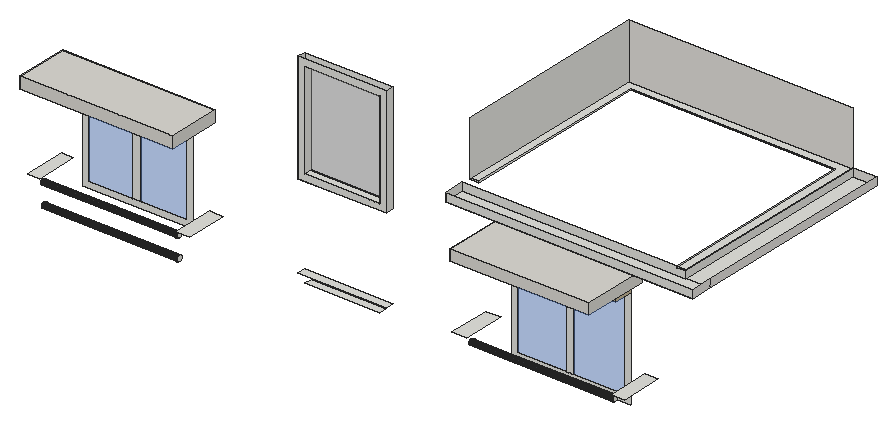
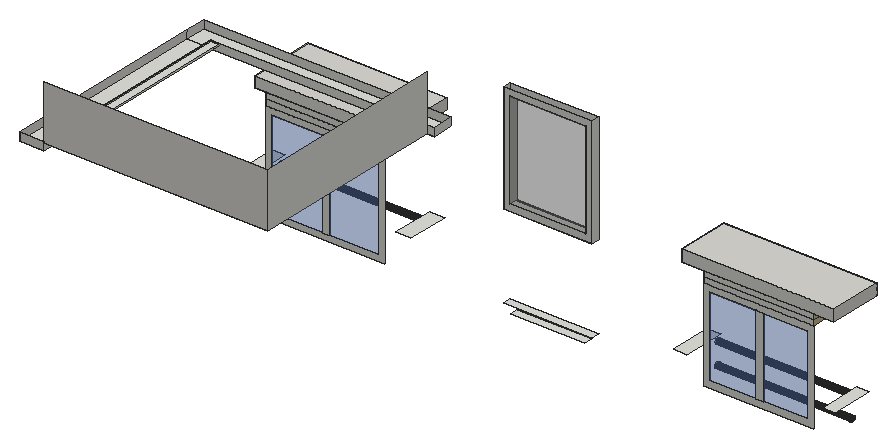
# SketchUp Ruby script. Lengths in inches.
U = 1.inch
M = Sketchup.active_model
def pt(a) = Geom::Point3d.new(a.map { |v| v * U })
def face(e, loops, mat)
  f = e.add_face(loops[0].map { |a| pt(a) })
  loops[1..].each { |l| e.add_face(l.map { |a| pt(a) }).erase! }
  f.material = f.back_material = mat if mat
  f
end
# faces: each face lists its corners as indices into pts; further lists are holes
def faces(e, pts, list, mat = nil) = list.each { |f| face(e, (f[0].is_a?(Array) ? f : [f]).map { |l| l.map { |i| pts[i] } }, mat) }
# xy, xz, yz: faces in a plane at the given z, y or x. An outline is a flat list of corners, or four numbers for a rectangle; further outlines are holes
def ring(l) = l.size == 4 ? [[l[0], l[1]], [l[2], l[1]], [l[2], l[3]], [l[0], l[3]]] : l.each_slice(2).to_a
def flat(e, list, mat, &to3) = list.each { |f| face(e, (f[0].is_a?(Array) ? f : [f]).map { |l| ring(l).map { |u, v| to3.(u, v) } }, mat) }
def xy(e, z, list, mat = nil) = flat(e, list, mat) { |x, y| [x, y, z] }
def xz(e, y, list, mat = nil) = flat(e, list, mat) { |x, z| [x, y, z] }
def yz(e, x, list, mat = nil) = flat(e, list, mat) { |y, z| [x, y, z] }
def lines(e, pts, list) = list.each { |a, b| e.add_line(pt(pts[a]), pt(pts[b])) }
# prism: a flat outline (further loops are holes) pulled along v
def prism(e, loops, v, mat = nil)
  f = face(e, loops, mat); d = Geom::Vector3d.new(v.map { |x| x * U })
  f.pushpull(f.normal.samedirection?(d) ? d.length : -d.length)
end
def box(e, o, s, mat = nil) = prism(e, [[o, [o[0] + s[0], o[1], o[2]], [o[0] + s[0], o[1] + s[1], o[2]], [o[0], o[1] + s[1], o[2]]]], [0, 0, s[2]], mat)
def at(x, y, z, deg = 0) = Geom::Transformation.translation(pt([x, y, z])) * Geom::Transformation.rotation(ORIGIN, Z_AXIS, deg.degrees)
def axes(o, x, y, z) = Geom::Transformation.new([*x, 0, *y, 0, *z, 0, *pt(o).to_a, 1])
def part(name) = M.definitions.add(name)
# library, detail: a bought-in or finely detailed component or shape, given as its bounding box
def library(name, o, s) = part(name).tap { |d| box(d.entities, o, s) }
def detail(e, o, s) = box(e.add_group.entities, o, s)
def put(e, d, t, mat = nil) = e.add_instance(d, t).tap { |i| i.material = mat if mat }
def group(e, t, mat = nil) = e.add_group.tap { |g| g.transformation = t; g.material = mat if mat }.entities
root = M.entities
M.materials.add("[Color M07]").color = [58, 58, 58]
M.materials.add("[Formica Laminate Dark]").color = [50, 53, 60]
M.materials.add("[Quartz Light Brown]").color = [199, 184, 152]
M.materials.add("[Terrazzo Tile Accent]").color = [224, 221, 217]
M.materials.add("[Terrazzo Tile Light]").color = [219, 217, 210]
M.materials.add("[Translucent Glass Blue]").color = [85, 126, 201]
M.materials["[Translucent Glass Blue]"].alpha = 0.5
M.materials.add("[Translucent Glass Gray]").color = [128, 128, 128]
M.materials["[Translucent Glass Gray]"].alpha = 0.5
xy(root,492.32,[[183.4,109.54,226.8,114.1]])
xy(root,496.3125,[[179.41,109.54,230.79,114.1]])
xy(root,503.49,[[103.3,91.47,103.56,91.5,103.8,91.6,104.01,91.76,104.16,91.97,104.26,92.21,104.3,92.47,104.26,92.73,104.16,92.97,104.01,93.18,103.8,93.33,103.56,93.43,103.3,93.47,103.04,93.43,102.8,93.33,102.59,93.18,102.43,92.97,102.33,92.73,102.3,92.47,102.33,92.21,102.43,91.97,102.59,91.76,102.8,91.6,103.04,91.5]])
xy(root,503.62,[[67.24,91.47,67.49,91.5,67.74,91.6,67.94,91.76,68.1,91.97,68.2,92.21,68.24,92.47,68.2,92.73,68.1,92.97,67.94,93.18,67.74,93.33,67.49,93.43,67.24,93.47,66.98,93.43,66.74,93.33,66.53,93.18,66.37,92.97,66.27,92.73,66.24,92.47,66.27,92.21,66.37,91.97,66.53,91.76,66.74,91.6,66.98,91.5]])
xy(root,504.05,[[108.86,91.47,109.12,91.5,109.36,91.6,109.57,91.76,109.73,91.97,109.83,92.21,109.86,92.47,109.83,92.73,109.73,92.97,109.57,93.18,109.36,93.33,109.12,93.43,108.86,93.47,108.6,93.43,108.36,93.33,108.15,93.18,107.99,92.97,107.89,92.73,107.86,92.47,107.89,92.21,107.99,91.97,108.15,91.76,108.36,91.6,108.6,91.5]])
xy(root,504.12,[[72.86,91.47,73.12,91.5,73.36,91.6,73.57,91.76,73.73,91.97,73.83,92.21,73.86,92.47,73.83,92.73,73.73,92.97,73.57,93.18,73.36,93.33,73.12,93.43,72.86,93.47,72.6,93.43,72.36,93.33,72.15,93.18,71.99,92.97,71.89,92.73,71.86,92.47,71.89,92.21,71.99,91.97,72.15,91.76,72.36,91.6,72.6,91.5]])
xy(root,504.18,[[78.17,91.47,78.43,91.5,78.67,91.6,78.88,91.76,79.04,91.97,79.14,92.21,79.17,92.47,79.14,92.73,79.04,92.97,78.88,93.18,78.67,93.33,78.43,93.43,78.17,93.47,77.91,93.43,77.67,93.33,77.47,93.18,77.31,92.97,77.21,92.73,77.17,92.47,77.21,92.21,77.31,91.97,77.47,91.76,77.67,91.6,77.91,91.5]])
xy(root,504.3,[[61.92,91.47,62.18,91.5,62.42,91.6,62.63,91.76,62.79,91.97,62.89,92.21,62.92,92.47,62.89,92.73,62.79,92.97,62.63,93.18,62.42,93.33,62.18,93.43,61.92,93.47,61.66,93.43,61.42,93.33,61.22,93.18,61.06,92.97,60.96,92.73,60.92,92.47,60.96,92.21,61.06,91.97,61.22,91.76,61.42,91.6,61.66,91.5]])
xy(root,504.43,[[97.92,91.47,98.18,91.5,98.42,91.6,98.63,91.76,98.79,91.97,98.89,92.21,98.92,92.47,98.89,92.73,98.79,92.97,98.63,93.18,98.42,93.33,98.18,93.43,97.92,93.47,97.66,93.43,97.42,93.33,97.22,93.18,97.06,92.97,96.96,92.73,96.92,92.47,96.96,92.21,97.06,91.97,97.22,91.76,97.42,91.6,97.66,91.5]])
xy(root,504.49,[[52.05,91.47,52.31,91.5,52.55,91.6,52.76,91.76,52.91,91.97,53.01,92.21,53.05,92.47,53.01,92.73,52.91,92.97,52.76,93.18,52.55,93.33,52.31,93.43,52.05,93.47,51.79,93.43,51.55,93.33,51.34,93.18,51.18,92.97,51.08,92.73,51.05,92.47,51.08,92.21,51.18,91.97,51.34,91.76,51.55,91.6,51.79,91.5]])
xy(root,504.67,[[92.55,91.47,92.81,91.5,93.05,91.6,93.26,91.76,93.41,91.97,93.51,92.21,93.55,92.47,93.51,92.73,93.41,92.97,93.26,93.18,93.05,93.33,92.81,93.43,92.55,93.47,92.29,93.43,92.05,93.33,91.84,93.18,91.68,92.97,91.58,92.73,91.55,92.47,91.58,92.21,91.68,91.97,91.84,91.76,92.05,91.6,92.29,91.5],[115.11,91.47,115.37,91.5,115.61,91.6,115.82,91.76,115.98,91.97,116.08,92.21,116.11,92.47,116.08,92.73,115.98,92.97,115.82,93.18,115.61,93.33,115.37,93.43,115.11,93.47,114.85,93.43,114.61,93.33,114.4,93.18,114.24,92.97,114.14,92.73,114.11,92.47,114.14,92.21,114.24,91.97,114.4,91.76,114.61,91.6,114.85,91.5],[120.49,91.47,120.74,91.5,120.99,91.6,121.19,91.76,121.35,91.97,121.45,92.21,121.49,92.47,121.45,92.73,121.35,92.97,121.19,93.18,120.99,93.33,120.74,93.43,120.49,93.47,120.23,93.43,119.99,93.33,119.78,93.18,119.62,92.97,119.52,92.73,119.49,92.47,119.52,92.21,119.62,91.97,119.78,91.76,119.99,91.6,120.23,91.5]])
xy(root,504.8,[[84.85,90.875,85.25,90.93,85.625,91.08,85.95,91.33,86.2,91.66,86.35,92.03,86.41,92.4375,86.35,92.84,86.2,93.22,85.95,93.54,85.625,93.79,85.25,93.95,84.85,94,84.44,93.95,84.0625,93.79,83.74,93.54,83.49,93.22,83.34,92.84,83.28,92.4375,83.34,92.03,83.49,91.66,83.74,91.33,84.0625,91.08,84.44,90.93]])
xy(root,505.01,[[47.49,91.47,47.74,91.5,47.99,91.6,48.19,91.76,48.35,91.97,48.45,92.21,48.49,92.47,48.45,92.73,48.35,92.97,48.19,93.18,47.99,93.33,47.85,93.39,47.12,93.39,46.99,93.33,46.78,93.18,46.62,92.97,46.52,92.73,46.49,92.47,46.52,92.21,46.62,91.97,46.78,91.76,46.99,91.6,47.23,91.5],[56.74,91.47,56.99,91.5,57.24,91.6,57.44,91.76,57.6,91.97,57.7,92.21,57.74,92.47,57.7,92.73,57.6,92.97,57.44,93.18,57.24,93.33,57.1,93.39,56.37,93.39,56.24,93.33,56.03,93.18,55.87,92.97,55.77,92.73,55.74,92.47,55.77,92.21,55.87,91.97,56.03,91.76,56.24,91.6,56.48,91.5],[47.12,93.39,47.85,93.39,47.74,93.43,47.49,93.47,47.23,93.43],[56.37,93.39,57.1,93.39,56.99,93.43,56.74,93.47,56.48,93.43]])
xy(root,506.99,[[38.09,89.73,44.94,114.1],[124.21,89.73,132.15,114.1]])
xy(root,507.16,[[359.09,91.9,359.32,91.93,359.53,92.02,359.71,92.16,359.85,92.34,359.9375,92.55,359.97,92.78,359.9375,93.01,359.85,93.22,359.71,93.4,359.53,93.54,359.32,93.625,359.09,93.65,358.86,93.625,358.65,93.54,358.47,93.4,358.33,93.22,358.25,93.01,358.22,92.78,358.25,92.55,358.33,92.34,358.47,92.16,358.65,92.02,358.86,91.93]])
xy(root,507.22,[[300.4,91.9,300.63,91.93,300.84,92.02,301.02,92.16,301.16,92.34,301.25,92.55,301.28,92.78,301.25,93.01,301.16,93.22,301.02,93.4,300.84,93.54,300.63,93.625,300.4,93.65,300.18,93.625,299.97,93.54,299.78,93.4,299.65,93.22,299.56,93.01,299.53,92.78,299.56,92.55,299.65,92.34,299.78,92.16,299.97,92.02,300.18,91.93]])
xy(root,507.41,[[305.59,91.9,305.82,91.93,306.03,92.02,306.21,92.16,306.35,92.34,306.4375,92.55,306.47,92.78,306.4375,93.01,306.35,93.22,306.21,93.4,306.03,93.54,305.82,93.625,305.59,93.65,305.36,93.625,305.15,93.54,304.97,93.4,304.83,93.22,304.75,93.01,304.72,92.78,304.75,92.55,304.83,92.34,304.97,92.16,305.15,92.02,305.36,91.93],[354.15,91.9,354.38,91.93,354.59,92.02,354.77,92.16,354.91,92.34,355,92.55,355.03,92.78,355,93.01,354.91,93.22,354.77,93.4,354.59,93.54,354.38,93.625,354.15,93.65,353.93,93.625,353.72,93.54,353.53,93.4,353.4,93.22,353.31,93.01,353.28,92.78,353.31,92.55,353.4,92.34,353.53,92.16,353.72,92.02,353.93,91.93]])
xy(root,507.47,[[295.4,91.9,295.63,91.93,295.84,92.02,296.02,92.16,296.16,92.34,296.25,92.55,296.28,92.78,296.25,93.01,296.16,93.22,296.02,93.4,295.84,93.54,295.63,93.625,295.4,93.65,295.18,93.625,294.97,93.54,294.78,93.4,294.65,93.22,294.56,93.01,294.53,92.78,294.56,92.55,294.65,92.34,294.78,92.16,294.97,92.02,295.18,91.93],[310.97,91.9,311.19,91.93,311.4,92.02,311.58,92.16,311.72,92.34,311.8125,92.55,311.84,92.78,311.8125,93.01,311.72,93.22,311.58,93.4,311.4,93.54,311.19,93.625,310.97,93.65,310.74,93.625,310.53,93.54,310.35,93.4,310.21,93.22,310.12,93.01,310.09,92.78,310.12,92.55,310.21,92.34,310.35,92.16,310.53,92.02,310.74,91.93]])
xy(root,507.54,[[368.53,91.9,368.75,91.93,368.97,92.02,369.15,92.16,369.29,92.34,369.375,92.55,369.4,92.78,369.375,93.01,369.29,93.22,369.15,93.4,368.97,93.54,368.75,93.625,368.53,93.65,368.3,93.625,368.09,93.54,367.91,93.4,367.77,93.22,367.68,93.01,367.65,92.78,367.68,92.55,367.77,92.34,367.91,92.16,368.09,92.02,368.3,91.93]])
xy(root,507.6,[[373.47,91.9,373.69,91.93,373.9,92.02,374.08,92.16,374.22,92.34,374.3125,92.55,374.34,92.78,374.3125,93.01,374.22,93.22,374.08,93.4,373.9,93.54,373.69,93.625,373.47,93.65,373.24,93.625,373.03,93.54,372.85,93.4,372.71,93.22,372.62,93.01,372.59,92.78,372.62,92.55,372.71,92.34,372.85,92.16,373.03,92.02,373.24,91.93]])
xy(root,507.81,[[335.9,91.32,336.3,91.37,336.68,91.53,337,91.78,337.25,92.1,337.41,92.48,337.46,92.88,337.41,93.28,337.25,93.66,337,93.99,336.71,94.21,335.08,94.21,334.79,93.99,334.54,93.66,334.39,93.28,334.33,92.88,334.39,92.48,334.54,92.1,334.79,91.78,335.11,91.53,335.49,91.37],[324.9,91.9,325.13,91.93,325.34,92.02,325.52,92.16,325.66,92.34,325.75,92.55,325.78,92.78,325.75,93.01,325.66,93.22,325.52,93.4,325.34,93.54,325.13,93.625,324.9,93.65,324.68,93.625,324.47,93.54,324.28,93.4,324.15,93.22,324.06,93.01,324.03,92.78,324.06,92.55,324.15,92.34,324.28,92.16,324.47,92.02,324.68,91.93],[335.08,94.21,336.71,94.21,336.68,94.23,336.3,94.39,335.9,94.44,335.49,94.39,335.11,94.23]])
xy(root,507.91,[[363.65,91.9,363.88,91.93,364.09,92.02,364.27,92.16,364.41,92.34,364.5,92.55,364.53,92.78,364.5,93.01,364.41,93.22,364.27,93.4,364.09,93.54,363.88,93.625,363.65,93.65,363.43,93.625,363.22,93.54,363.03,93.4,362.9,93.22,362.81,93.01,362.78,92.78,362.81,92.55,362.9,92.34,363.03,92.16,363.22,92.02,363.43,91.93]])
xy(root,508.19,[[317.9,91.9,318.13,91.93,318.34,92.02,318.52,92.16,318.66,92.34,318.75,92.55,318.78,92.78,318.75,93.01,318.66,93.22,318.52,93.4,318.34,93.54,318.13,93.625,317.9,93.65,317.68,93.625,317.47,93.54,317.28,93.4,317.15,93.22,317.06,93.01,317.03,92.78,317.06,92.55,317.15,92.34,317.28,92.16,317.47,92.02,317.68,91.93],[330.28,91.9,330.5,91.93,330.72,92.02,330.9,92.16,331.04,92.34,331.125,92.55,331.15,92.78,331.125,93.01,331.04,93.22,330.9,93.4,330.72,93.54,330.5,93.625,330.28,93.65,330.05,93.625,329.84,93.54,329.66,93.4,329.52,93.22,329.43,93.01,329.4,92.78,329.43,92.55,329.52,92.34,329.66,92.16,329.84,92.02,330.05,91.93],[343.53,91.9,343.75,91.93,343.97,92.02,344.15,92.16,344.29,92.34,344.375,92.55,344.4,92.78,344.375,93.01,344.29,93.22,344.15,93.4,343.97,93.54,343.75,93.625,343.53,93.65,343.3,93.625,343.09,93.54,342.91,93.4,342.77,93.22,342.68,93.01,342.65,92.78,342.68,92.55,342.77,92.34,342.91,92.16,343.09,92.02,343.3,91.93]])
xy(root,508.56,[[349.09,91.9,349.32,91.93,349.53,92.02,349.71,92.16,349.85,92.34,349.9375,92.55,349.97,92.78,349.9375,93.01,349.85,93.22,349.71,93.4,349.53,93.54,349.32,93.625,349.09,93.65,348.86,93.625,348.65,93.54,348.47,93.4,348.33,93.22,348.25,93.01,348.22,92.78,348.25,92.55,348.33,92.34,348.47,92.16,348.65,92.02,348.86,91.93]])
xy(root,511.22,[[284.68,89.73,293.32,114.1],[377.32,89.73,384.86,114.1]])
xy(root,545.4375,[[179.41,109.54,230.79,114.1]])
xy(root,547.64,[[50.46,105.98,114.59,114.1]],"[Quartz Light Brown]")
xy(root,549.11,[[183.08,109.54,227.11,114.1]])
xy(root,550.63,[[299.93,102.85,369.18,114.1]],"[Quartz Light Brown]")
xy(root,550.85,[[50.46,108.04,114.59,114.1]])
xy(root,550.85,[[50.46,105.98,114.59,108.04]],"[Quartz Light Brown]")
xy(root,554.07,[[50.05,85.59,50.42,85.64,50.46,85.66,50.46,88.4,50.42,88.42,50.05,88.47,49.68,88.42,49.33,88.28,49.03,88.05,48.81,87.75,48.66,87.4,48.61,87.03,48.66,86.66,48.81,86.3125,49.03,86.02,49.33,85.79,49.68,85.64],[50.46,85.66,50.77,85.79,51.07,86.02,51.3,86.3125,51.4375,86.66,51.49,87.03,51.4375,87.4,51.3,87.75,51.07,88.05,50.77,88.28,50.46,88.4],[50.46,108.04,114.59,114.1]])
xy(root,554.07,[[38.67,83.48,38.67,114.1,50.46,114.1,50.46,88.4,50.42,88.42,50.05,88.47,49.68,88.42,49.33,88.28,49.03,88.05,48.81,87.75,48.66,87.4,48.61,87.03,48.66,86.66,48.81,86.3125,49.03,86.02,49.33,85.79,49.68,85.64,50.05,85.59,50.42,85.64,50.46,85.66,50.46,83.48],[50.46,83.48,50.46,85.66,50.77,85.79,51.07,86.02,51.3,86.3125,51.4375,86.66,51.49,87.03,51.4375,87.4,51.3,87.75,51.07,88.05,50.77,88.28,50.46,88.4,50.46,108.04,114.59,108.04,114.59,83.48],[[114.59,83.48,127.48,114.1],[119.6875,84.95,120.06,85,120.4,85.14,120.7,85.37,120.93,85.67,121.07,86.02,121.125,86.39,121.07,86.76,120.93,87.11,120.7,87.4,120.4,87.63,120.06,87.78,119.6875,87.82,119.3125,87.78,118.97,87.63,118.67,87.4,118.44,87.11,118.3,86.76,118.25,86.39,118.3,86.02,118.44,85.67,118.67,85.37,118.97,85.14,119.3125,85]]],"[Terrazzo Tile Light]")
xy(root,554.17,[[299.93,107.35,369.18,114.1]])
xy(root,554.17,[[299.93,102.85,369.18,107.35]],"[Quartz Light Brown]")
xy(root,557.7,[[299.93,107.35,369.18,114.1]])
xy(root,557.86,[[[294.48,75.67,375.23,114.1],[300.64,84.97,301.01,85.02,301.36,85.17,301.65,85.4,301.88,85.69,302.03,86.04,302.07,86.41,302.03,86.78,301.88,87.13,301.65,87.43,301.36,87.66,301.01,87.8,300.64,87.85,300.26,87.8,299.92,87.66,299.62,87.43,299.39,87.13,299.25,86.78,299.2,86.41,299.25,86.04,299.39,85.69,299.62,85.4,299.92,85.17,300.26,85.02],[368.82,84.97,369.2,85.02,369.54,85.17,369.84,85.4,370.07,85.69,370.21,86.04,370.26,86.41,370.21,86.78,370.07,87.13,369.84,87.43,369.54,87.66,369.2,87.8,368.82,87.85,368.45,87.8,368.11,87.66,367.81,87.43,367.58,87.13,367.4375,86.78,367.39,86.41,367.4375,86.04,367.58,85.69,367.81,85.4,368.11,85.17,368.45,85.02]]],"[Terrazzo Tile Light]")
xy(root,560.89,[[38.67,83.48,127.48,114.1]],"[Terrazzo Tile Light]")
xy(root,564.11,[[294.48,75.67,375.23,114.1]],"[Terrazzo Tile Light]")
xy(root,569,[[270.97,102.04,415.04,114.1],[401.16,114.1,415.04,235.11]])
xy(root,573,[[395.61,114.1,395.61,229.56,276.53,229.56,276.53,119.66,270.97,119.66,270.97,235.11,401.16,235.11,401.16,114.1]])
xz(root,75.67,[[294.48,557.86,375.23,564.11]],"[Terrazzo Tile Light]")
xz(root,83.48,[[38.67,554.07,127.48,560.89]],"[Terrazzo Tile Light]")
xz(root,102.04,[[270.97,569,415.04,573.6875]])
xz(root,102.85,[[299.93,550.63,369.18,554.17]],"[Quartz Light Brown]")
xz(root,105.98,[[50.46,547.64,114.59,550.85]],"[Quartz Light Brown]")
xz(root,107.35,[[299.93,554.17,369.18,557.7]],"[Quartz Light Brown]")
xz(root,108.04,[[50.46,550.85,114.59,554.07]],"[Quartz Light Brown]")
xz(root,109.54,[[[179.41,545.4375,230.79,609.125],[183.08,549.11,227.11,605.45]]])
xz(root,114.1,[[[299.93,492.45,369.18,550.63],[303.53,496.05,365.57,547.03]],[[50.46,494.26,114.59,547.64],[54.09,497.89,110.95,544]],[331.78,496.05,335.88,547.03],[79.63,497.89,84.26,544],[[179.41,545.4375,230.79,609.125],[183.08,549.11,227.11,605.45]],
  [50.46,547.64,114.59,550.85],[299.93,550.63,369.18,554.17],[50.46,550.85,114.59,554.07],[38.67,554.07,127.48,560.89],[299.93,554.17,369.18,557.7],
  [294.48,557.86,375.23,564.11],[270.97,569,270.97,573.6875,395.61,573.6875,395.61,573,401.16,573,401.16,569],[395.61,573,401.16,573.6875]])
xz(root,114.1,[[303.53,496.05,331.78,547.03],[335.88,496.05,365.57,547.03],[54.09,497.89,79.63,544],[84.26,497.89,110.95,544]],"[Translucent Glass Blue]")
xz(root,114.1,[[183.08,549.11,227.11,605.45]],"[Translucent Glass Gray]")
xz(root,119.66,[[270.97,573,276.53,573.6875]])
xz(root,229.56,[[276.53,573,395.61,573.6875]])
xz(root,235.11,[[401.16,569,415.04,573.6875],[270.97,573,401.16,604.875]],"[Terrazzo Tile Accent]")
yz(root,38.67,[[83.48,554.07,114.1,560.89]],"[Terrazzo Tile Light]")
yz(root,50.46,[[105.98,547.64,114.1,550.85],[108.04,550.85,114.1,554.07]],"[Quartz Light Brown]")
yz(root,114.59,[[105.98,547.64,114.1,550.85],[108.04,550.85,114.1,554.07]],"[Quartz Light Brown]")
yz(root,124.21,[[92.45,490.42,92.84,490.47,93.2,490.62,93.51,490.86,93.75,491.17,93.9,491.53,93.95,491.92,93.9,492.31,93.75,492.67,93.51,492.98,93.2,493.22,92.84,493.37,92.45,493.42,92.06,493.37,91.7,493.22,91.39,492.98,91.15,492.67,91,492.31,90.95,491.92,91,491.53,91.15,491.17,91.39,490.86,91.7,490.62,92.06,490.47],[92.15,502.86,92.52,502.91,92.87,503.05,93.16,503.28,93.39,503.58,93.53,503.92,93.58,504.3,93.53,504.67,93.39,505.01,93.16,505.3125,92.87,505.54,92.52,505.68,92.15,505.73,91.77,505.68,91.43,505.54,91.13,505.3125,90.9,505.01,90.76,504.67,90.71,504.3,90.76,503.92,90.9,503.58,91.13,503.28,91.43,503.05,91.77,502.91]])
yz(root,127.48,[[83.48,554.07,114.1,560.89]],"[Terrazzo Tile Light]")
yz(root,179.41,[[109.54,545.4375,114.1,609.125]])
yz(root,183.08,[[109.54,549.11,114.1,605.45]])
yz(root,227.11,[[109.54,549.11,114.1,605.45]])
yz(root,230.79,[[109.54,545.4375,114.1,609.125]])
yz(root,270.97,[[102.04,569,114.1,573.6875],[119.66,573,235.11,604.875]])
yz(root,276.53,[[119.66,573,229.56,573.6875]])
yz(root,294.48,[[75.67,557.86,114.1,564.11]],"[Terrazzo Tile Light]")
yz(root,299.93,[[102.85,550.63,114.1,554.17],[107.35,554.17,114.1,557.7]],"[Quartz Light Brown]")
yz(root,369.18,[[102.85,550.63,114.1,554.17],[107.35,554.17,114.1,557.7]],"[Quartz Light Brown]")
yz(root,375.23,[[75.67,557.86,114.1,564.11]],"[Terrazzo Tile Light]")
yz(root,377.32,[[92.71,506.31,93.09,506.36,93.46,506.51,93.77,506.74,94.01,507.06,94.16,507.42,94.21,507.81,94.16,508.19,94.01,508.56,93.77,508.87,93.46,509.1,93.09,509.25,92.71,509.31,92.32,509.25,91.96,509.1,91.65,508.87,91.41,508.56,91.26,508.19,91.21,507.81,91.26,507.42,91.41,507.06,91.65,506.74,91.96,506.51,92.32,506.36]])
yz(root,395.61,[[114.1,573,119.66,573.6875],[119.66,573,229.56,573.6875]])
yz(root,401.16,[[114.1,569,235.11,573],[114.1,573,235.11,573.6875]])
yz(root,415.04,[[102.04,569,114.1,573.6875],[114.1,569,235.11,573.6875]],"[Terrazzo Tile Accent]")
p = [[124.21,92.45,490.42],[124.21,92.06,490.47],[44.94,92.06,490.47],[44.94,92.45,490.42],[124.21,92.84,490.47],[44.94,92.84,490.47],
  [124.21,91.7,490.62],[44.94,91.7,490.62],[124.21,93.2,490.62],[44.94,93.2,490.62],[124.21,91.39,490.86],[44.94,91.39,490.86],
  [124.21,93.51,490.86],[44.94,93.51,490.86],[124.21,91.15,491.17],[44.94,91.15,491.17],[124.21,93.75,491.17],[44.94,93.75,491.17],
  [124.21,91,491.53],[44.94,91,491.53],[124.21,93.9,491.53],[44.94,93.9,491.53],[124.21,90.95,491.92],[44.94,90.95,491.92],
  [124.21,93.95,491.92],[44.94,93.95,491.92],[84.44,93.95,491.92],[85.25,93.95,491.92],[124.21,91,492.31],[44.94,91,492.31],
  [124.21,93.9,492.31],[44.94,93.9,492.31],[124.21,91.15,492.67],[44.94,91.15,492.67],[124.21,93.75,492.67],[44.94,93.75,492.67],
  [124.21,91.39,492.98],[44.94,91.39,492.98],[124.21,93.51,492.98],[44.94,93.51,492.98],[124.21,91.7,493.22],[44.94,91.7,493.22],
  [124.21,93.2,493.22],[44.94,93.2,493.22],[124.21,92.06,493.37],[44.94,92.06,493.37],[124.21,92.84,493.37],[44.94,92.84,493.37],
  [124.21,92.45,493.42],[44.94,92.45,493.42],[124.21,91.77,502.91],[124.21,91.43,503.05],[44.94,91.43,503.05],[44.94,91.77,502.91],
  [124.21,92.15,502.86],[44.94,92.15,502.86],[124.21,92.52,502.91],[44.94,92.52,502.91],[124.21,92.87,503.05],[44.94,92.87,503.05],
  [124.21,91.13,503.28],[44.94,91.13,503.28],[124.21,93.16,503.28],[44.94,93.16,503.28],[124.21,90.9,503.58],[44.94,90.9,503.58],
  [124.21,93.39,503.58],[44.94,93.39,503.58],[124.21,90.76,503.92],[44.94,90.76,503.92],[124.21,93.53,503.92],[44.94,93.53,503.92],
  [124.21,90.71,504.3],[44.94,90.71,504.3],[124.21,93.58,504.3],[44.94,93.58,504.3],[124.21,90.76,504.67],[44.94,90.76,504.67],
  [124.21,93.53,504.67],[44.94,93.53,504.67],[124.21,90.9,505.01],[44.94,90.9,505.01],[124.21,93.39,505.01],[44.94,93.39,505.01],
  [47.12,93.39,505.01],[47.85,93.39,505.01],[56.37,93.39,505.01],[57.1,93.39,505.01],[124.21,91.13,505.3125],[44.94,91.13,505.3125],
  [124.21,93.16,505.3125],[44.94,93.16,505.3125],[124.21,91.43,505.54],[44.94,91.43,505.54],[124.21,92.87,505.54],[44.94,92.87,505.54],
  [124.21,91.77,505.68],[44.94,91.77,505.68],[124.21,92.52,505.68],[44.94,92.52,505.68],[124.21,92.15,505.73],[44.94,92.15,505.73],
  [377.32,92.71,506.31],[377.32,92.32,506.36],[293.32,92.32,506.36],[293.32,92.71,506.31],[377.32,93.09,506.36],[293.32,93.09,506.36],
  [377.32,91.96,506.51],[293.32,91.96,506.51],[377.32,93.46,506.51],[293.32,93.46,506.51],[377.32,91.65,506.74],[293.32,91.65,506.74],
  [377.32,93.77,506.74],[293.32,93.77,506.74],[377.32,91.41,507.06],[293.32,91.41,507.06],[377.32,94.01,507.06],[293.32,94.01,507.06],
  [377.32,91.26,507.42],[293.32,91.26,507.42],[377.32,94.16,507.42],[293.32,94.16,507.42],[377.32,91.21,507.81],[293.32,91.21,507.81],
  [377.32,94.21,507.81],[293.32,94.21,507.81],[335.08,94.21,507.81],[336.71,94.21,507.81],[377.32,91.26,508.19],[293.32,91.26,508.19],
  [377.32,94.16,508.19],[293.32,94.16,508.19],[377.32,91.41,508.56],[293.32,91.41,508.56],[377.32,94.01,508.56],[293.32,94.01,508.56],
  [377.32,91.65,508.87],[293.32,91.65,508.87],[377.32,93.77,508.87],[293.32,93.77,508.87],[377.32,91.96,509.1],[293.32,91.96,509.1],
  [377.32,93.46,509.1],[293.32,93.46,509.1],[377.32,92.32,509.25],[293.32,92.32,509.25],[377.32,93.09,509.25],[293.32,93.09,509.25],
  [377.32,92.71,509.31],[293.32,92.71,509.31]]
faces(root,p,[[0,1,2,3],[4,0,3,5],[1,6,7,2],[8,4,5,9],[6,10,11,7],[12,8,9,13],[10,14,15,11],[16,12,13,17],
  [14,18,19,15],[20,16,17,21],[18,22,23,19],[24,20,21,25,26,27],[22,28,29,23],[30,24,27,26,25,31],[28,32,33,29],[34,30,31,35],
  [32,36,37,33],[38,34,35,39],[36,40,41,37],[42,38,39,43],[40,44,45,41],[46,42,43,47],[44,48,49,45],[48,46,47,49],
  [50,51,52,53],[54,50,53,55],[56,54,55,57],[58,56,57,59],[51,60,61,52],[62,58,59,63],[60,64,65,61],[66,62,63,67],
  [64,68,69,65],[70,66,67,71],[68,72,73,69],[74,70,71,75],[72,76,77,73],[78,74,75,79],[76,80,81,77],[82,78,79,83,84,85,86,87],
  [80,88,89,81],[90,82,87,86,85,84,83,91],[88,92,93,89],[94,90,91,95],[92,96,97,93],[98,94,95,99],[96,100,101,97],[100,98,99,101]],"[Color M07]")
faces(root,p,[[102,103,104,105],[106,102,105,107],[103,108,109,104],[110,106,107,111],[108,112,113,109],[114,110,111,115],[112,116,117,113],[118,114,115,119],
  [116,120,121,117],[122,118,119,123],[120,124,125,121],[126,122,123,127,128,129],[124,130,131,125],[132,126,129,128,127,133],[130,134,135,131],[136,132,133,137],
  [134,138,139,135],[140,136,137,141],[138,142,143,139],[144,140,141,145],[142,146,147,143],[148,144,145,149],[146,150,151,147],[150,148,149,151]],"[Formica Laminate Dark]")
